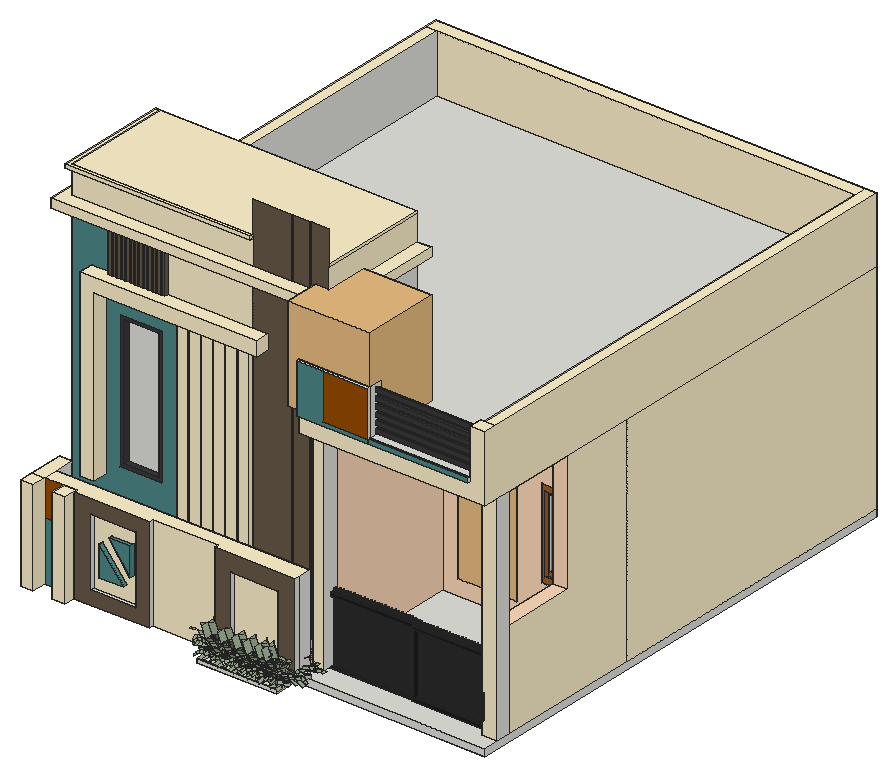
# SketchUp Ruby script. Lengths in inches.
U = 1.inch
M = Sketchup.active_model
def pt(a) = Geom::Point3d.new(a.map { |v| v * U })
def face(e, loops, mat)
  f = e.add_face(loops[0].map { |a| pt(a) })
  loops[1..].each { |l| e.add_face(l.map { |a| pt(a) }).erase! }
  f.material = f.back_material = mat if mat
  f
end
# faces: each face lists its corners as indices into pts; further lists are holes
def faces(e, pts, list, mat = nil) = list.each { |f| face(e, (f[0].is_a?(Array) ? f : [f]).map { |l| l.map { |i| pts[i] } }, mat) }
# xy, xz, yz: faces in a plane at the given z, y or x. An outline is a flat list of corners, or four numbers for a rectangle; further outlines are holes
def ring(l) = l.size == 4 ? [[l[0], l[1]], [l[2], l[1]], [l[2], l[3]], [l[0], l[3]]] : l.each_slice(2).to_a
def flat(e, list, mat, &to3) = list.each { |f| face(e, (f[0].is_a?(Array) ? f : [f]).map { |l| ring(l).map { |u, v| to3.(u, v) } }, mat) }
def xy(e, z, list, mat = nil) = flat(e, list, mat) { |x, y| [x, y, z] }
def xz(e, y, list, mat = nil) = flat(e, list, mat) { |x, z| [x, y, z] }
def yz(e, x, list, mat = nil) = flat(e, list, mat) { |y, z| [x, y, z] }
def lines(e, pts, list) = list.each { |a, b| e.add_line(pt(pts[a]), pt(pts[b])) }
# prism: a flat outline (further loops are holes) pulled along v
def prism(e, loops, v, mat = nil)
  f = face(e, loops, mat); d = Geom::Vector3d.new(v.map { |x| x * U })
  f.pushpull(f.normal.samedirection?(d) ? d.length : -d.length)
end
def box(e, o, s, mat = nil) = prism(e, [[o, [o[0] + s[0], o[1], o[2]], [o[0] + s[0], o[1] + s[1], o[2]], [o[0], o[1] + s[1], o[2]]]], [0, 0, s[2]], mat)
def at(x, y, z, deg = 0) = Geom::Transformation.translation(pt([x, y, z])) * Geom::Transformation.rotation(ORIGIN, Z_AXIS, deg.degrees)
def axes(o, x, y, z) = Geom::Transformation.new([*x, 0, *y, 0, *z, 0, *pt(o).to_a, 1])
def part(name) = M.definitions.add(name)
# library, detail: a bought-in or finely detailed component or shape, given as its bounding box
def library(name, o, s) = part(name).tap { |d| box(d.entities, o, s) }
def detail(e, o, s) = box(e.add_group.entities, o, s)
def put(e, d, t, mat = nil) = e.add_instance(d, t).tap { |i| i.material = mat if mat }
def group(e, t, mat = nil) = e.add_group.tap { |g| g.transformation = t; g.material = mat if mat }.entities
root = M.entities
M.materials.add("[Color C01]").color = [255, 219, 186]
M.materials.add("[Color C07]").color = [104, 89, 74]
M.materials.add("[Color C07]1").color = [153, 76, 0]
M.materials.add("[Color D01]").color = [255, 242, 204]
M.materials.add("[Color H08]").color = [77, 137, 137]
M.materials.add("[Color M07]").color = [58, 58, 58]
M.materials.add("[Color M08]").color = [30, 30, 30]
M.materials.add("[Translucent_Glass_Safety]").color = [204, 235, 244]
M.materials["[Translucent_Glass_Safety]"].alpha = 0.5
M.materials.add("[Translucent_Glass_Sky_Reflection]").color = [125, 138, 183]
M.materials["[Translucent_Glass_Sky_Reflection]"].alpha = 0.52
M.materials.add("[Wood Square Tile 01]").color = [164, 91, 44]
M.materials.add("[Wood Square Tile 02]").color = [160, 95, 34]
M.materials.add("hymenocallis littoralis").color = [156, 172, 146]
c1 = part("Group\#428")
prism(c1.entities,[[[0,1.97,0],[0,1.97,1.18],[0,0,1.18],[0,0,0]],[[0,1.92,1.13],[0,1.92,0.05],[0,0.05,0.05],[0,0.05,1.13]]],[98.43,0,0])
c2 = part("Group\#430")
xy(c2.entities,0,[[0.3,0,0.22,0.01,0.15,0.04,0.09,0.09,0.04,0.15,0.01,0.22,0,0.3,0.3,0.3],[0.3,0,0.3,0.3,0.59,0.3,0.58,0.22,0.55,0.15,0.5,0.09,0.44,0.04,0.37,0.01],[0,0.3,0.01,0.37,0.04,0.44,0.09,0.5,0.15,0.55,0.22,0.58,0.3,0.59,0.3,0.3],[0.3,0.3,0.3,0.59,0.37,0.58,0.44,0.55,0.5,0.5,0.55,0.44,0.58,0.37,0.59,0.3]])
xy(c2.entities,39.37,[[0.3,0,0.37,0.01,0.44,0.04,0.5,0.09,0.55,0.15,0.58,0.22,0.59,0.3,0.58,0.37,0.55,0.44,0.5,0.5,0.44,0.55,0.37,0.58,0.3,0.59,0.22,0.58,0.15,0.55,0.09,0.5,0.04,0.44,0.01,0.37,0,0.3,0.01,0.22,0.04,0.15,0.09,0.09,0.15,0.04,0.22,0.01]])
p = [[0.09,0.09,0],[0.15,0.04,0],[0.15,0.04,39.37],[0.09,0.09,39.37],[0.22,0.01,0],[0.22,0.01,39.37],
  [0.3,0,0],[0.3,0,39.37],[0.37,0.01,0],[0.37,0.01,39.37],[0.44,0.04,0],[0.44,0.04,39.37],
  [0.5,0.09,0],[0.5,0.09,39.37],[0.01,0.22,0],[0.04,0.15,0],[0.04,0.15,39.37],[0.01,0.22,39.37],
  [0.55,0.15,0],[0.55,0.15,39.37],[0.58,0.22,0],[0.58,0.22,39.37],[0,0.3,0],[0,0.3,39.37],
  [0.59,0.3,0],[0.59,0.3,39.37],[0.01,0.37,0],[0.01,0.37,39.37],[0.58,0.37,0],[0.58,0.37,39.37],
  [0.09,0.5,0],[0.04,0.44,0],[0.04,0.44,39.37],[0.09,0.5,39.37],[0.55,0.44,0],[0.5,0.5,0],
  [0.5,0.5,39.37],[0.55,0.44,39.37],[0.15,0.55,0],[0.15,0.55,39.37],[0.44,0.55,0],[0.44,0.55,39.37],
  [0.22,0.58,0],[0.22,0.58,39.37],[0.3,0.59,0],[0.3,0.59,39.37],[0.37,0.58,0],[0.37,0.58,39.37]]
faces(c2.entities,p,[[0,1,2,3],[1,4,5,2],[4,6,7,5],[6,8,9,7],[8,10,11,9],[10,12,13,11],[14,15,16,17],[15,0,3,16],
  [12,18,19,13],[18,20,21,19],[22,14,17,23],[20,24,25,21],[26,22,23,27],[24,28,29,25],[30,31,32,33],[31,26,27,32],
  [34,35,36,37],[28,34,37,29],[38,30,33,39],[35,40,41,36],[42,38,39,43],[44,42,43,45],[46,44,45,47],[40,46,47,41]])
c3 = part("Group\#429")
prism(c3.entities,[[[0.01,0.22,35.83],[0,0.3,35.83],[0.01,0.37,35.83],[0.04,0.44,35.83],[0.09,0.5,35.83],[0.15,0.55,35.83],[0.22,0.58,35.83],[0.3,0.59,35.83],[0.37,0.58,35.83],[0.44,0.55,35.83],[0.5,0.5,35.83],[0.55,0.44,35.83],[0.58,0.37,35.83],[0.59,0.3,35.83],[0.58,0.22,35.83],[0.55,0.15,35.83],[0.5,0.09,35.83],[0.44,0.04,35.83],[0.37,0.01,35.83],[0.3,0,35.83],[0.22,0.01,35.83],[0.15,0.04,35.83],[0.09,0.09,35.83],[0.04,0.15,35.83]]],[0,0,3.54])
c4 = part("Metal railing panel")
g1 = group(c4.entities,at(0,0,0))
put(g1,c1,axes([0,0,39.76],[1,0,0],[0,0,-1],[0,1,0]),"[Color M08]")
put(g1,c1,axes([0,0,1.97],[1,0,0],[0,0,-1],[0,1,0]),"[Color M08]")
put(g1,c1,axes([98.43,0,37.8],[0,0,-0.364],[-1,0,0],[0,1,0]),"[Color M08]")
put(g1,c1,axes([1.97,0,37.8],[0,0,-0.364],[-1,0,0],[0,1,0]),"[Color M08]")
g2 = group(c4.entities,at(1.67,0.3,1.97))
put(g2,c2,at(78.74,0,0),"[Color M08]")
put(g2,c2,at(90.55,0,0),"[Color M08]")
put(g2,c2,at(82.68,0,0),"[Color M08]")
put(g2,c2,at(86.61,0,0),"[Color M08]")
put(g2,c2,at(66.93,0,0),"[Color M08]")
put(g2,c2,at(11.8125,0,0),"[Color M08]")
put(g2,c2,at(15.75,0,0),"[Color M08]")
put(g2,c2,at(47.24,0,0),"[Color M08]")
put(g2,c2,at(59.06,0,0),"[Color M08]")
put(g2,c3,at(0,0,0),"[Color M08]")
put(g2,c2,at(39.37,0,0),"[Color M08]")
put(g2,c2,at(62.99,0,0),"[Color M08]")
put(g2,c2,at(55.12,0,0),"[Color M08]")
put(g2,c2,at(19.69,0,0),"[Color M08]")
put(g2,c2,at(35.43,0,0),"[Color M08]")
put(g2,c2,at(7.875,0,0),"[Color M08]")
put(g2,c2,at(23.62,0,0),"[Color M08]")
put(g2,c2,at(31.5,0,0),"[Color M08]")
put(g2,c2,at(43.31,0,0),"[Color M08]")
put(g2,c2,at(27.56,0,0),"[Color M08]")
put(g2,c2,at(3.9375,0,0),"[Color M08]")
put(g2,c2,at(51.18,0,0),"[Color M08]")
put(g2,c2,at(70.87,0,0),"[Color M08]")
put(g2,c2,at(74.8,0,0),"[Color M08]")
put(g2,c3,at(94.49,0,0),"[Color M08]")
c5 = part("Sliding window")
xy(c5.entities,0,[[0,0,4.33,55.51]])
xy(c5.entities,2.76,[[0,2.76,2,27.76],[0,27.76,0.82,52.76],[0.82,27.76,2.36,52.76]])
xy(c5.entities,2.76,[[3.15,2.76,4.33,27.76]],"[Wood Square Tile 01]")
xy(c5.entities,2.76,[[2.36,27.76,4.33,52.76]],"[Wood Square Tile 02]")
xy(c5.entities,4.72,[[2,4.72,2.4,26.38],[2.76,4.72,3.15,26.38],[0.82,29.13,1.22,50.79],[1.97,29.13,2.36,50.79]])
xy(c5.entities,36.61,[[2,4.72,2.4,26.38],[2.76,4.72,3.15,26.38],[0.82,29.13,1.22,50.79],[1.97,29.13,2.36,50.79]])
xy(c5.entities,38.58,[[0,2.76,2,27.76],[0,27.76,0.82,52.76],[0.82,27.76,2.36,52.76]])
xy(c5.entities,38.58,[[3.15,2.76,4.33,27.76],[2.36,27.76,4.33,52.76]],"[Wood Square Tile 01]")
xy(c5.entities,41.34,[[0,0,4.33,55.51]])
xz(c5.entities,0,[[0,0,4.33,41.34]])
xz(c5.entities,2.76,[[0,2.76,2,38.58]])
xz(c5.entities,2.76,[[3.15,2.76,4.33,38.58]],"[Wood Square Tile 01]")
xz(c5.entities,4.72,[[2,4.72,2.4,36.61],[2.76,4.72,3.15,36.61]])
xz(c5.entities,26.38,[[2,4.72,2.4,36.61],[2.76,4.72,3.15,36.61]])
xz(c5.entities,27.76,[[0.82,2.76,2,38.58],[2,2.76,2.36,38.58],[2.36,2.76,3.15,38.58]])
xz(c5.entities,29.13,[[0.82,4.72,1.22,36.61],[1.97,4.72,2.36,36.61]])
xz(c5.entities,50.79,[[0.82,4.72,1.22,36.61],[1.97,4.72,2.36,36.61]])
xz(c5.entities,52.76,[[0,2.76,0.82,38.58],[0.82,2.76,2.36,38.58]])
xz(c5.entities,52.76,[[2.36,2.76,4.33,38.58]],"[Wood Square Tile 01]")
xz(c5.entities,55.51,[[0,0,4.33,41.34]])
yz(c5.entities,0,[[[0,0,55.51,41.34],[2.76,2.76,52.76,38.58]]])
yz(c5.entities,0.82,[[[27.76,2.76,52.76,38.58],[29.13,4.72,50.79,36.61]]])
yz(c5.entities,1.22,[[29.13,4.72,50.79,36.61]],"[Translucent_Glass_Sky_Reflection]")
yz(c5.entities,1.97,[[29.13,4.72,50.79,36.61]],"[Translucent_Glass_Sky_Reflection]")
yz(c5.entities,2,[[[2.76,2.76,27.76,38.58],[4.72,4.72,26.38,36.61]]])
yz(c5.entities,2.36,[[[27.76,2.76,52.76,38.58],[29.13,4.72,50.79,36.61]]],"[Wood Square Tile 02]")
yz(c5.entities,2.4,[[4.72,4.72,26.38,36.61]],"[Translucent_Glass_Safety]")
yz(c5.entities,2.76,[[4.72,4.72,26.38,36.61]],"[Translucent_Glass_Safety]")
yz(c5.entities,3.15,[[[2.76,2.76,27.76,38.58],[4.72,4.72,26.38,36.61]]],"[Wood Square Tile 02]")
yz(c5.entities,4.33,[[[0,0,55.51,41.34],[2.76,2.76,52.76,38.58]]],"[Wood Square Tile 02]")
c6 = library("door2",[0,0,0],[35.42,7.875,78.74])
c7 = part("Group\#856")
xy(c7.entities,7.38,[[0,0,5.5,15.91]],"hymenocallis littoralis")
p = [[5.5,28.78,0],[5.5,26.79,3.44],[0,26.79,3.44],[0,28.78,0],[0,23.75,6],[5.5,23.75,6],
  [0,15.91,7.38],[5.5,15.91,7.38]]
faces(c7.entities,p,[[0,1,2,3],[4,2,1,5],[6,4,5,7]],"hymenocallis littoralis")
c8 = part("Group\#854")
xy(c8.entities,7.38,[[0,0,5.5,15.91],[0,15.91,5.5,23.87]],"hymenocallis littoralis")
p = [[5.5,31.07,4.3],[5.5,27.74,6.47],[0,27.74,6.47],[0,31.07,4.3],[0,23.87,7.38],[5.5,23.87,7.38]]
faces(c8.entities,p,[[0,1,2,3],[4,2,1,5]],"hymenocallis littoralis")
c9 = part("Group\#857")
xy(c9.entities,7.38,[[0,0,5.6,15.91]],"hymenocallis littoralis")
p = [[5.6,28.78,0],[5.6,26.79,3.44],[0,26.79,3.44],[0,28.78,0],[0,23.75,6],[5.6,23.75,6],
  [0,15.91,7.38],[5.6,15.91,7.38]]
faces(c9.entities,p,[[0,1,2,3],[4,2,1,5],[6,4,5,7]],"hymenocallis littoralis")
c10 = part("Group\#855")
put(c10.entities,c8,axes([6.09,8.57,-0.52],[0.446,0.85617,0.26089],[-0.18444,-0.19731,0.96283],[0.87582,-0.47754,0.0699]))
put(c10.entities,c8,axes([6.29,7.28,-1.71],[0.37058,0.92707,-0.05667],[-0.32382,0.19004,0.99128],[0.87712,-0.32925,0.34964]))
put(c10.entities,c8,axes([11.04,16.14,-0.7],[1,0,0],[0,0.16628,1.02662],[0,-1.18456,0.19186]))
c11 = part("Group\#860")
put(c11.entities,c7,axes([24.57,32.05,-1.76],[0.9552,-0.22102,-0.19681],[0.4036,0.95545,0.88585],[-0.00568,-0.67859,0.7345]))
put(c11.entities,c7,axes([23.95,29.24,-2.4],[0,1,0],[-0.76041,0,0.64945],[0.64945,0,0.76041]))
put(c11.entities,c7,axes([24.22,24.72,-0.48],[-0.70711,0.70711,0],[-0.32757,-0.32757,0.80237],[0.61237,0.61237,0.5]))
put(c11.entities,c8,axes([20.66,37.22,-0.63],[1.12361,0.03262,0.39091],[-0.43499,0.29739,0.78777],[0.09852,-1.27434,0.37535]))
put(c11.entities,c7,axes([28.75,24.45,-2.4],[-1,0,0],[0,-0.76041,0.64945],[0,0.64945,0.76041]))
put(c11.entities,c9,axes([30.4,30.98,-3.7],[0.65676,-0.72002,0.22414],[0.55667,0.66341,0.5],[-0.50871,-0.20361,0.83652]))
put(c11.entities,c9,axes([32.41,29.61,-3.7],[0.04029,-0.97372,0.22414],[0.85287,0.15038,0.5],[-0.52057,0.17102,0.83652]))
put(c11.entities,c7,axes([31.89,25.85,-1.76],[-0.92056,0.33739,-0.19681],[-0.5186,-0.89824,0.88585],[0.08952,0.67268,0.7345]))
put(c11.entities,c7,axes([25.55,34.78,-0.48],[0.86603,0.5,0],[-0.25,0.43301,0.86603],[0.43301,-0.75,0.5]))
put(c11.entities,c9,axes([20.4,16.9375,-8.07],[-0.70711,0.70711,0],[-0.35754,-0.35754,0.65422],[1.3987,1.3987,1.52882]))
put(c11.entities,c7,axes([32.86,34.14,-0.48],[0.76604,-0.64279,0],[0.32139,0.38302,0.86603],[-0.55667,-0.66341,0.5]))
put(c11.entities,c7,axes([27.15,34.7,-0.1],[0.82472,-0.17528,-0.53769],[0.53769,0.53769,0.64945],[0.17528,-0.82472,0.53769]))
put(c11.entities,c7,axes([33.58,28.77,-2.4],[0,-1,0],[0.76041,0,0.64945],[-0.64945,0,0.76041]))
put(c11.entities,c7,axes([26.43,23.87,-2.81],[-0.75126,0.04415,0.65853],[0.53769,-0.53769,0.64945],[0.38276,0.84199,0.3802]))
put(c11.entities,c7,axes([28.78,23.98,-2.4],[-1,0,0],[0,-0.76041,0.64945],[0,0.64945,0.76041]))
put(c11.entities,c7,axes([25.39,25.38,-2.4],[-0.70711,0.70711,0],[-0.53769,-0.53769,0.64945],[0.45923,0.45923,0.76041]))
put(c11.entities,c7,axes([27.32,21.63,-0.1],[-0.45923,0.70711,-0.53769],[-0.76041,0,0.64945],[0.45923,0.70711,0.53769]))
put(c11.entities,c7,axes([25.17,27.625,-1.76],[0.56416,0.80187,-0.19681],[-0.66673,0.66673,0.80532],[0.62659,-0.26057,0.7345]))
put(c11.entities,c9,axes([27.59,27.04,-3.96],[-0.8993,-0.06127,0.43301],[0.2962,-0.8138,0.5],[0.32175,0.57791,0.75]))
put(c11.entities,c9,axes([26.98,24.5,-3.18],[-0.5,0.86603,0],[-0.75,-0.43301,0.5],[0.43301,0.25,0.86603]))
put(c11.entities,c9,axes([24.55,27.74,-3.7],[0.29517,0.92878,0.22414],[-0.85287,0.15038,0.5],[0.43068,-0.33875,0.83652]))
put(c11.entities,c9,axes([24.26,29.8,-3.18],[0.76604,0.64279,0],[-0.47317,0.5639,0.425],[0.32139,-0.38302,0.86603]))
put(c11.entities,c9,axes([25.98,32.46,-3.18],[1,0,0],[0,0.86603,0.5],[0,-0.5,0.86603]))
put(c11.entities,c7,axes([28.78,33.57,-2.4],[1,0,0],[0,0.76041,0.64945],[0,-0.64945,0.76041]))
put(c11.entities,c10,at(14.99,21.38,2.5))
put(c11.entities,c8,axes([34.63,26.34,-1.46],[-0.70089,-0.70877,0.07994],[0.4756,-0.38088,0.79293],[-0.53156,0.59378,0.60405]))
put(c11.entities,c8,axes([28.14,16.92,1.8125],[-1.19719,0.6912,0],[-0.09607,-0.16641,0.94244],[0.68444,1.18549,0.17613]))
put(c11.entities,c8,axes([31.5625,35.84,0.97],[0.66765,-1.1564,0.35779],[0.04445,0.30732,0.91033],[-1.20828,-0.64496,0.17012]))
put(c11.entities,c8,axes([38.94,22.51,0.89],[-0.97932,-0.67164,-0.05202],[0.27787,-0.41401,0.90999],[-0.85985,0.93577,0.32097]))
put(c11.entities,c8,axes([38.44,21.09,1.98],[-1.02864,-0.54856,0.2395],[0.33481,0.06999,0.88388],[-0.77261,1.08328,0.06417]))
put(c11.entities,c9,axes([35.02,30.51,-1.3],[-0.17365,-0.98481,0],[0.60224,-0.10619,0.79122],[-0.7792,0.13739,0.61153]))
put(c11.entities,c9,axes([29.41,22.33,-1.3],[-0.93969,0.34202,0],[-0.20915,-0.57465,0.79122],[0.27061,0.74351,0.61153]))
put(c11.entities,c8,axes([19.64,36,-1.62],[1.18194,0.09546,0.08234],[-0.14377,0.68823,0.76313],[0.21457,-1.1326,0.62386]))
put(c11.entities,c9,axes([24.25,24.14,-1.3],[-0.34202,0.93969,0],[-0.57465,-0.20915,0.79122],[0.74351,0.27061,0.61153]))
put(c11.entities,c9,axes([25.98,34.61,-1.3],[1,0,0],[0,0.61153,0.79122],[0,-0.79122,0.61153]))
put(c11.entities,c9,axes([31.16,34.41,-1.64],[0.56518,-0.80224,-0.19234],[0.73413,0.34233,0.72935],[-0.47639,-0.50772,0.71782]))
put(c11.entities,c9,axes([40.52,26.84,-5.82],[-0.42262,-0.90631,0],[0.48019,-0.22391,0.68552],[-1.43418,0.66877,1.22305]))
put(c11.entities,c7,axes([29.86,38.42,-1.01],[0.89064,-0.37013,0.26413],[-0.03924,0.63286,1.01918],[-0.45353,-0.76487,0.45748]))
put(c11.entities,c7,axes([29.34,22.4,-0.48],[-0.99619,-0.08716,0],[0.04358,-0.4981,0.86603],[-0.07548,0.86273,0.5]))
c12 = part("Group\#858")
xz(c12.entities,10.07,[[9.07,0,10.07,31.01],[0,31.01,0,45.12,20.13,45.12,20.13,31.01,10.07,31.01,10.07,32.58,9.07,32.58,9.07,31.01]],"hymenocallis littoralis")
yz(c12.entities,10.07,[[0,31.01,20.13,45.12]],"hymenocallis littoralis")
p = [[9.57,9.2,0],[10.07,10.07,0],[10.07,10.07,31.01],[10.07,10.07,32.58],[9.57,9.2,32.58]]
faces(c12.entities,p,[[0,1,2,3,4]],"hymenocallis littoralis")
c13 = part("cây lá nắng")
put(c13.entities,c11,axes([49.26,-2.75,0],[0.63109,0.63109,0],[-0.63109,0.63109,0],[0,0,0.935]))
g3 = group(c13.entities,at(26.6,-8.68,0))
put(g3,c7,axes([-4.72,35.73,-1.65],[0.74231,0.46334,-0.18402],[-0.34827,0.85768,0.82827],[0.42467,-0.43184,0.68675]))
put(g3,c7,axes([-3.34,33.57,-2.24],[-0.63109,0.63109,0],[-0.47989,-0.47989,0.60723],[0.40986,0.40986,0.71098]))
put(g3,c7,axes([-0.3125,30.89,-0.45],[-0.8925,0,0],[0,-0.41345,0.75022],[0,0.77293,0.4675]))
put(g3,c8,axes([-10.79,39.66,-0.59],[0.68852,0.72969,0.3655],[-0.4622,-0.08684,0.73657],[0.86641,-0.74205,0.35095]))
put(g3,c7,axes([2.71,33.57,-2.24],[-0.63109,-0.63109,0],[0.47989,-0.47989,0.60723],[-0.40986,0.40986,0.71098]))
put(g3,c9,axes([-0.37,38.74,-3.46],[0.86887,-0.03992,0.20957],[-0.06737,0.76999,0.4675],[-0.19255,-0.44954,0.78214]))
put(g3,c9,axes([1.76,39.14,-3.46],[0.63993,-0.58908,0.20957],[0.44333,0.63315,0.4675],[-0.43646,-0.2206,0.78214]))
put(g3,c7,axes([3.81,36.4375,-1.65],[-0.79389,-0.36803,-0.18402],[0.23959,-0.89415,0.82827],[-0.36803,0.48102,0.68675]))
put(g3,c7,axes([-5.83,38.07,-0.45],[0.231,0.86209,0],[-0.43104,0.1155,0.80973],[0.74659,-0.20005,0.4675]))
put(g3,c9,axes([2.18,23.5625,-7.55],[-0.8925,0,0],[0,-0.45128,0.6117],[0,1.76542,1.42944]))
put(g3,c7,axes([-0.8125,42.28,-0.45],[0.8891,0.07779,0],[-0.03889,0.44455,0.80973],[0.06737,-0.76999,0.4675]))
put(g3,c7,axes([-4.76,39.03,-0.09],[0.63109,0.40986,-0.50274],[0,0.67866,0.60723],[0.63109,-0.40986,0.50274]))
put(g3,c7,axes([3.03,39.35,-2.24],[0.63109,-0.63109,0],[0.47989,0.47989,0.60723],[-0.40986,-0.40986,0.71098]))
put(g3,c7,axes([1.61,31.74,-2.625],[-0.50198,-0.44625,0.61573],[0.67866,0,0.60723],[-0.28982,0.77293,0.35549]))
put(g3,c7,axes([3.03,33.3,-2.24],[-0.63109,-0.63109,0],[0.47989,-0.47989,0.60723],[-0.40986,0.40986,0.71098]))
put(g3,c7,axes([0.01,32.04,-2.24],[-0.8925,0,0],[0,-0.67866,0.60723],[0,0.57963,0.71098]))
put(g3,c7,axes([3.59,30.89,-0.09],[-0.73607,0.15643,-0.50274],[-0.47989,-0.47989,0.60723],[-0.15643,0.73607,0.50274]))
put(g3,c7,axes([-1.55,33.32,-1.65],[-0.15002,0.86209,-0.18402],[-0.84154,0,0.75297],[0.55988,0.231,0.68675]))
put(g3,c9,axes([0.35,34.48,-3.71],[-0.52887,-0.60621,0.40487],[0.70051,-0.32665,0.4675],[-0.16166,0.56777,0.70125]))
put(g3,c9,axes([2.61,39.13,-1.74],[-0.86209,0.231,0],[-0.23031,-0.85954,0.15531],[0.03162,0.11799,0.91645]))
put(g3,c9,axes([-2.02,33,-3.46],[-0.39986,0.77243,0.20957],[-0.63315,-0.44333,0.4675],[0.48558,0.05802,0.78214]))
put(g3,c9,axes([-3.49,34.12,-2.97],[0.07779,0.8891,0],[-0.65449,0.05726,0.39737],[0.44455,-0.03889,0.80973]))
put(g3,c9,axes([-4.09,36.88,-2.97],[0.63109,0.63109,0],[-0.54654,0.54654,0.4675],[0.31555,-0.31555,0.80973]))
put(g3,c7,axes([-3.02,39.35,-2.24],[0.63109,0.63109,0],[-0.47989,0.47989,0.60723],[0.40986,-0.40986,0.71098]))
put(g3,c10,axes([-4.03,22.95,2.33],[0.63109,0.63109,0],[-0.63109,0.63109,0],[0,0,0.935]))
put(g3,c8,axes([5.24,38.48,-1.37],[0.00497,-0.88963,0.07474],[0.54052,0.05978,0.74139],[-0.71019,0.03927,0.56479]))
put(g3,c8,axes([7.08,28.4375,1.7],[-1.19175,-0.31933,0],[0.04439,-0.16565,0.88118],[-0.31621,1.1801,0.16468]))
put(g3,c8,axes([-2.7,42.54,0.91],[1.15114,-0.30845,0.33454],[-0.1659,0.22199,0.85115],[-0.3555,-1.16957,0.15907]))
put(g3,c8,axes([10.37,38.78,0.83],[-0.19417,-1.04191,-0.04864],[0.43664,-0.08592,0.85084],[-1.1332,0.04791,0.30011]))
put(g3,c8,axes([10.95,37.5625,1.85],[-0.30298,-0.99536,0.22393],[0.16713,0.25547,0.82643],[-1.17124,0.19607,0.06]))
put(g3,c9,axes([2.84,41.36,-1.22],[0.51192,-0.73109,0],[0.44708,0.31305,0.73979],[-0.57846,-0.40504,0.57178]))
put(g3,c9,axes([4.47,32.65,-1.22],[-0.80888,-0.37719,0],[0.23066,-0.49465,0.73979],[-0.29844,0.64,0.57178]))
put(g3,c8,axes([-10.32,35.12,-1.51],[0.68567,0.80616,0.07699],[-0.52507,0.3436,0.71352],[0.85019,-0.57936,0.58331]))
put(g3,c9,axes([0.07,30.54,-1.22],[-0.80888,0.37719,0],[-0.23066,-0.49465,0.73979],[0.29844,0.64,0.57178]))
put(g3,c9,axes([-5.45,38.24,-1.22],[0.63109,0.63109,0],[-0.38593,0.38593,0.73979],[0.49934,-0.49934,0.57178]))
put(g3,c9,axes([-2.05,41.38,-1.53],[0.86296,-0.14961,-0.17984],[0.24726,0.67935,0.68194],[0.01977,-0.62107,0.67116]))
put(g3,c9,axes([8.63,42.51,-5.4375],[0.30525,-0.83868,0],[0.44435,0.16173,0.64096],[-1.32716,-0.48305,1.14356]))
put(g3,c7,axes([-5.4,43.09,-0.94],[0.79566,0.32849,0.24696],[-0.42416,0.37462,0.95293],[0.19648,-0.76892,0.42774]))
put(g3,c7,axes([4.38,32.65,-0.45],[-0.57369,-0.68369,0],[0.34185,-0.28684,0.80973],[-0.5921,0.49683,0.4675]))
put(g3,c9,axes([-2,33.84,-0.15],[-0.24601,0.85793,0],[-0.85539,-0.24528,0.15531],[0.11742,0.03367,0.91645]))
put(g3,c9,axes([0.17,30.83,-4.47],[-0.24601,0.85793,0],[-0.85539,-0.24528,0.15531],[0.11742,0.03367,0.91645]))
put(g3,c9,axes([-1.97,32.18,-4.47],[0.58524,0.67383,0],[-0.67184,0.58351,0.15531],[0.09222,-0.0801,0.91645]))
put(g3,c9,axes([-2,34.71,-4.47],[0.88392,-0.12346,0],[0.12309,0.88131,0.15531],[-0.0169,-0.12098,0.91645]))
put(g3,c9,axes([0.11,36.12,-4.47],[0.37822,-0.8084,0],[0.80601,0.37711,0.15531],[-0.11064,-0.05177,0.91645]))
put(c13.entities,c12,axes([29.71,14.29,6.94],[0.425,0.73612,0],[-0.6771,0.39092,-0.33349],[-0.26859,0.15507,0.72712]))
put(c13.entities,c12,axes([42.0625,26.12,6.94],[0.85,0,0],[0,0.78185,-0.33349],[0,0.33349,0.78185]))
put(c13.entities,c11,axes([7.3125,23.0625,0],[0.8925,0,0],[0,0.8925,0],[0,0,0.935]))
put(c13.entities,c12,axes([24.4375,40.23,2.05],[0.85,0,0],[0,0.85,0],[0,0,0.85]))
c14 = part("Planting+101")
put(c14.entities,c13,axes([21.34,32.96,-4.59],[0,-0.71,0],[-0.71,0,0],[0,0,0.71]))
c15 = library("Flora+17",[-57.52,158.6,-38.64],[66.99,62.88,77.28])
c16 = part("Group\#1")
xz(c16.entities,0,[[0,0,2.8125,38.62]])
yz(c16.entities,0,[[0,0,3,38.62]])
yz(c16.entities,2.8125,[[0,0,3,38.62]])
c17 = part("Group\#2")
p = [[0,0,0.02],[0,1.98,0],[81.3125,1.98,0],[81.3125,0,0.02],[0,0.12,3.625],[81.3125,0.12,3.625],
  [0,2.11,3.61],[81.3125,2.11,3.61]]
faces(c17.entities,p,[[0,1,2,3],[4,0,3,5],[1,6,7,2],[6,4,5,7]])
xy(root,0,[[150.35,2.54,150.35,21.8125,151.875,21.8125,151.875,4.0625,213.72,4.0625,213.72,19.97,215.25,19.97,215.25,2.54],[151.875,4.0625,213.72,18.4375],[0,9.8125,10.625,21.8125],[26.125,9.8125,36.75,21.8125],[36.75,18.4375,36.75,21.8125,0,21.8125,0,49.6875,10.625,49.6875,10.625,421.6875,370.625,421.6875,370.625,21.8125,217.88,21.8125,217.88,19.97,151.875,19.97,151.875,21.8125,98.84,21.8125,98.84,18.4375],
  [151.875,18.4375,213.72,19.97]])
xy(root,2.4375,[[150.35,2.54,215.25,2.54,215.25,18.4375,213.72,18.4375,213.72,4.0625,151.875,4.0625,151.875,21.8125,150.35,21.8125],[213.72,18.4375,215.25,19.97],[215.25,18.4375,217.88,19.97]])
xy(root,6,[[217.88,21.8125,370.625,21.8125,370.625,33.85,358.42,33.85,358.42,166.35,220.5,166.35,220.5,49.6875,227.12,49.6875,227.12,36.0625,217.88,36.0625,217.88,49.6875,205.92,49.6875,205.92,49.99,205.0625,49.99,205.0625,49.6875,190.92,49.6875,190.92,49.99,190,49.99,190,49.6875,158.1875,49.6875,158.1875,49.99,157.79,49.99,157.79,46.6875,148.18,46.6875,148.18,49.99,147.78,49.99,147.78,46.6875,138.17,46.6875,138.17,49.99,137.77,49.99,137.77,46.6875,128.17,46.6875,128.17,49.99,127.77,49.99,127.77,46.6875,118.16,46.6875,118.16,49.99,117.76,49.99,117.76,46.6875,108.15,46.6875,108.15,49.99,107.75,49.99,107.75,46.6875,98.15,46.6875,98.15,49.99,97.75,49.99,97.75,49.6875,10.625,49.6875,10.625,33.52,217.88,33.52],[358.42,45.67,370.625,166.35]])
xy(root,11.33,[[50.83,18.4375,87.51,21.8125]])
xy(root,13.49,[[165.37,18.4375,203.85,21.8125]])
xy(root,18,[[232.5,166.35,280.5,182.35]])
xy(root,22.6875,[[57.52,18.4375,77.7,21.8125]],"[Color H08]")
xy(root,39.88,[[301.46,166.35,353.08,191.72]])
xy(root,54.51,[[65.13,18.4375,83.06,21.8125]],"[Color H08]")
xy(root,64.51,[[165.37,18.4375,200.1875,21.8125],[200.1875,18.4375,203.85,21.8125]])
xy(root,66.67,[[50.83,18.4375,87.51,21.8125]])
xy(root,78,[[26.3125,37.6875,38.11,49.6875]])
xy(root,78,[[0,9.8125,10.625,21.8125],[26.125,9.8125,36.75,21.8125],[36.75,18.4375,98.84,18.4375,98.84,21.8125,151.875,21.8125,151.875,18.4375,217.88,18.4375,217.88,33.52,10.625,33.52,10.625,21.8125,36.75,21.8125],[0,21.8125,10.625,49.6875]],"[Color D01]")
xy(root,85.5625,[[358.42,45.67,370.625,106.01]],"[Color C01]")
xy(root,90.54,[[52.42,49.6875,81.72,54.8125]],"[Color M07]")
xy(root,102,[[232.5,166.35,280.5,182.35]])
xy(root,112.7,[[301.46,166.35,353.08,191.72]])
xy(root,183.5625,[[217.88,21.8125,217.88,49.6875,220.5,49.6875,220.5,166.35,358.42,166.35,358.42,106.01,370.625,106.01,370.625,45.67,358.42,45.67,358.42,33.85,370.625,33.85,370.625,21.8125]],"[Color C01]")
xy(root,184.3125,[[217.88,36.0625,227.12,49.6875]])
xy(root,189.9375,[[227.62,32.9375,361.5625,32.9375,361.5625,411.0625,19.625,411.0625,19.625,139.5,220.5,139.5,220.5,60.625,227.62,60.625]])
xy(root,196.53,[[52.42,49.6875,81.72,54.8125]],"[Color M07]")
xy(root,196.64,[[217.88,19.69,276.48,21.8]])
xy(root,200.25,[[276.48,21.8125,357.8,32.9375]])
xy(root,215.64,[[38.11,37.6875,38.11,49.6875,97.75,49.6875,97.75,49.99,98.15,49.99,98.15,46.6875,107.75,46.6875,107.75,49.99,108.15,49.99,108.15,46.6875,117.76,46.6875,117.76,49.99,118.16,49.99,118.16,46.6875,127.77,46.6875,127.77,49.99,128.17,49.99,128.17,46.6875,137.77,46.6875,137.77,49.99,138.17,49.99,138.17,46.6875,147.78,46.6875,147.78,49.99,148.18,49.99,148.18,46.6875,157.79,46.6875,157.79,49.99,158.1875,49.99,158.1875,49.6875,170.9375,49.6875,170.9375,37.6875]],"[Color D01]")
xy(root,227.33,[[26.3125,37.6875,170.9375,37.6875,170.9375,49.6875,45.2,49.6875,45.2,46.6875,42.38,46.6875,42.38,49.6875,26.3125,49.6875]],"[Color D01]")
xy(root,237.5625,[[217.88,19.69,276.48,21.8]])
xy(root,237.5625,[[217.88,21.8125,276.48,21.8125,276.48,32.9375,227.62,32.9375,227.62,60.625,220.5,60.625,220.5,49.6875,217.88,49.6875],[357.8,21.8125,370.625,32.9375],[361.5625,32.9375,370.625,421.6875],[10.625,139.5,19.625,411.0625],[10.625,411.0625,361.5625,421.6875]],"[Color D01]")
xy(root,265.94,[[158.1875,37.6875,158.1875,49.6875,190,49.6875,190,49.99,190.92,49.99,190.92,49.6875,205.0625,49.6875,205.0625,49.99,205.92,49.99,205.92,49.6875,220.5,49.6875,220.5,139.5,232.5,139.5,232.5,37.6875]])
xy(root,265.94,[[2.625,37.6875,2.625,139.5,10.625,139.5,10.625,49.6875,42.38,49.6875,42.38,46.6875,45.2,46.6875,45.2,49.6875,158.1875,49.6875,158.1875,37.6875]],"[Color D01]")
xy(root,272.92,[[2.625,37.6875,232.5,37.6875,232.5,139.5,220.5,139.5,220.5,49.6875,205.92,49.6875,205.92,49.99,205.0625,49.99,205.0625,49.6875,190.92,49.6875,190.92,49.99,190,49.99,190,49.6875,10.625,49.6875,10.625,139.5,2.625,139.5]],"[Color D01]")
xy(root,292.71,[[7.25,46.6875,10.625,49.6875],[10.625,46.6875,158.1875,49.6875],[7.25,49.6875,10.625,139.5]],"[Color D01]")
xy(root,292.96,[[158.1875,50.875,220.5,139.5]])
xy(root,295.71,[[7.25,46.6875,158.1875,46.6875,158.1875,49.6875,10.625,49.6875,10.625,139.5,7.25,139.5],[10.625,49.6875,158.1875,49.6875,158.1875,50.875,220.5,50.875,220.5,139.5,10.625,139.5]],"[Color D01]")
xy(root,321.41,[[190,49.6875,190.92,49.99],[205.0625,49.6875,205.92,49.99]])
xz(root,2.54,[[150.35,0,215.25,2.4375]])
xz(root,4.0625,[[151.875,0,213.72,2.4375]])
xz(root,9.8125,[[0,0,10.625,78],[26.125,0,36.75,78]],"[Color D01]")
xz(root,18.4375,[[[36.75,0,98.84,78],[50.83,11.33,87.51,66.67]],[[151.875,0,213.72,0,213.72,2.4375,217.88,2.4375,217.88,78,151.875,78],[165.37,13.49,203.85,64.51]]],"[Color C07]")
xz(root,18.4375,[[57.52,22.6875,77.7,22.6875,57.52,47.2],[83.06,31.32,83.06,54.51,65.13,54.51]],"[Color H08]")
xz(root,19.69,[[239.3,200.23,276.48,237.5625]],"[Color C07]1")
xz(root,19.69,[[217.88,196.64,276.48,196.64,276.48,200.23,239.3,200.23,239.3,237.5625,217.88,237.5625]],"[Color H08]")
xz(root,19.97,[[213.72,0,215.25,2.4375],[215.25,0,217.88,2.4375]])
xz(root,21.8,[[217.88,196.64,276.48,200.23],[217.88,200.23,276.48,237.5625]])
xz(root,21.8125,[[0,0,10.625,78],[26.125,0,36.75,78],[217.88,0,370.625,6]])
xz(root,21.8125,[[10.625,48.75,26.125,78]],"[Color C07]1")
xz(root,21.8125,[[98.84,0,150.35,0,150.35,2.4375,151.875,2.4375,151.875,78,98.84,78],[[50.83,11.33,87.51,66.67],[57.52,22.6875,57.52,47.2,77.7,22.6875],[83.06,31.32,65.13,54.51,83.06,54.51]],[165.37,13.49,203.85,64.51],[217.88,183.5625,370.625,183.5625,370.625,237.5625,357.8,237.5625,357.8,200.25,276.48,200.25,276.48,237.5625,217.88,237.5625]],"[Color D01]")
xz(root,21.8125,[[10.625,0,26.125,48.75]],"[Color H08]")
xz(root,32.9375,[[227.62,189.9375,227.62,237.5625,276.48,237.5625,276.48,200.25,357.8,200.25,357.8,237.5625,361.5625,237.5625,361.5625,189.9375]])
xz(root,33.52,[[10.625,6,206.03,78],[206.03,6,217.88,78]])
xz(root,33.85,[[358.42,6,370.625,183.5625]],"[Color D01]")
xz(root,36.0625,[[217.88,6,227.12,184.3125]],"[Color D01]")
xz(root,37.6875,[[26.3125,78,38.11,78,38.11,215.64,170.9375,215.64,170.9375,227.33,26.3125,227.33],[2.625,265.94,232.5,272.92]],"[Color D01]")
xz(root,45.67,[[358.42,6,370.625,85.5625],[358.42,85.5625,370.625,183.5625]])
xz(root,46.6875,[[98.15,6,107.75,215.64],[108.15,6,117.76,215.64],[118.16,6,127.77,215.64],[128.17,6,137.77,215.64],[138.17,6,147.78,215.64],
  [148.18,6,157.79,215.64],[7.25,292.71,158.1875,295.71]],"[Color D01]")
xz(root,49.6875,[[0,0,10.625,6],[0,6,10.625,78],[220.5,6,220.5,183.5625,217.88,183.5625,217.88,184.3125,227.12,184.3125,227.12,6],[217.88,189.5625,220.5,237.5625],[45.2,227.33,88.24,265.94],
  [10.625,292.71,158.1875,295.71]])
xz(root,49.6875,[[158.1875,6,190,6,190,265.94,158.1875,265.94,158.1875,227.33,170.9375,227.33,170.9375,215.64,158.1875,215.64],[190.92,6,205.0625,265.94],[205.92,6,217.88,6,217.88,237.5625,220.5,237.5625,220.5,265.94,205.92,265.94],[158.1875,272.92,190,321.41],[190.92,272.92,205.0625,321.41],
  [205.92,272.92,220.5,321.41]],"[Color C07]")
xz(root,49.6875,[[88.24,227.33,158.1875,265.94],[10.625,272.92,158.1875,292.71]],"[Color D01]")
xz(root,49.6875,[[[10.625,6,97.75,6,97.75,215.64,38.11,215.64,38.11,78,26.3125,78,26.3125,227.33,42.38,227.33,42.38,265.94,10.625,265.94],[49.35,87.47,84.79,199.6]]],"[Color H08]")
xz(root,49.6875,[[[49.35,87.47,84.79,199.6],[52.42,90.54,81.72,196.53]]],"[Color M07]")
xz(root,49.99,[[97.75,6,98.15,215.64],[107.75,6,108.15,215.64],[117.76,6,118.16,215.64],[127.77,6,128.17,215.64],[137.77,6,138.17,215.64],
  [147.78,6,148.18,215.64],[157.79,6,158.1875,215.64],[190,6,190.92,265.94],[205.0625,6,205.92,265.94],[190,272.92,190.92,321.41],
  [205.0625,272.92,205.92,321.41]])
xz(root,50.875,[[158.1875,292.96,220.5,295.71]])
xz(root,54.8125,[[52.42,90.54,81.72,196.53]])
xz(root,60.625,[[220.5,189.9375,227.62,237.5625]])
xz(root,106.01,[[358.42,85.5625,370.625,183.5625]],"[Color C01]")
xz(root,139.5,[[19.625,189.9375,19.625,237.5625,10.625,237.5625,10.625,295.71,220.5,295.71,220.5,189.9375],[2.625,265.94,10.625,272.92],[220.5,265.94,232.5,272.92],[7.25,292.71,10.625,295.71]],"[Color D01]")
xz(root,166.35,[[[220.5,6,358.42,183.5625],[232.5,18,280.5,102],[301.46,39.88,353.08,112.7]]],"[Color C01]")
xz(root,182.35,[[232.5,18,280.5,102]])
xz(root,191.72,[[301.46,39.88,353.08,112.7]])
xz(root,411.0625,[[19.625,189.9375,361.5625,237.5625]],"[Color D01]")
xz(root,421.6875,[[10.625,0,370.625,183.5625],[10.625,183.5625,370.625,237.5625]],"[Color D01]")
yz(root,0,[[9.8125,0,21.8125,78],[21.8125,0,49.6875,78]],"[Color D01]")
yz(root,2.625,[[37.6875,265.94,139.5,272.92]],"[Color D01]")
yz(root,7.25,[[46.6875,292.71,139.5,295.71]],"[Color D01]")
yz(root,10.625,[[33.52,6,49.6875,78],[49.6875,292.71,139.5,295.71]])
yz(root,10.625,[[9.8125,0,21.8125,78],[49.6875,0,421.6875,183.5625],[49.6875,183.5625,49.6875,189.5625,139.5,189.5625,139.5,237.5625,421.6875,237.5625,421.6875,183.5625],[49.6875,189.5625,139.5,265.94],[49.6875,272.92,139.5,292.71]],"[Color D01]")
yz(root,19.625,[[139.5,189.9375,411.0625,237.5625]])
yz(root,26.125,[[9.8125,0,21.8125,78]])
yz(root,26.3125,[[37.6875,78,49.6875,227.33]],"[Color D01]")
yz(root,36.75,[[18.4375,0,21.8125,78]])
yz(root,36.75,[[9.8125,0,18.4375,78]],"[Color D01]")
yz(root,38.11,[[37.6875,78,49.6875,215.64]],"[Color D01]")
yz(root,50.83,[[18.4375,11.33,21.8125,66.67]])
yz(root,52.42,[[49.6875,90.54,54.8125,196.53]],"[Color M07]")
yz(root,57.52,[[18.4375,22.6875,21.8125,47.2]],"[Color H08]")
yz(root,81.72,[[49.6875,90.54,54.8125,196.53]],"[Color M07]")
yz(root,83.06,[[18.4375,31.32,21.8125,54.51]],"[Color H08]")
yz(root,87.51,[[18.4375,11.33,21.8125,66.67]])
yz(root,97.75,[[49.6875,6,49.99,215.64]])
yz(root,98.15,[[46.6875,6,49.99,215.64]],"[Color D01]")
yz(root,98.84,[[18.4375,0,21.8125,78]])
yz(root,107.75,[[46.6875,6,49.99,215.64]])
yz(root,108.15,[[46.6875,6,49.99,215.64]])
yz(root,117.76,[[46.6875,6,49.99,215.64]])
yz(root,118.16,[[46.6875,6,49.99,215.64]])
yz(root,127.77,[[46.6875,6,49.99,215.64]])
yz(root,128.17,[[46.6875,6,49.99,215.64]])
yz(root,137.77,[[46.6875,6,49.99,215.64]])
yz(root,138.17,[[46.6875,6,49.99,215.64]])
yz(root,147.78,[[46.6875,6,49.99,215.64]])
yz(root,148.18,[[46.6875,6,49.99,215.64]])
yz(root,150.35,[[2.54,0,21.8125,2.4375]])
yz(root,151.875,[[4.0625,0,18.4375,2.4375],[18.4375,0,21.8125,2.4375],[18.4375,2.4375,21.8125,78]])
yz(root,157.79,[[46.6875,6,49.99,215.64]],"[Color D01]")
yz(root,158.1875,[[49.6875,6,49.99,215.64],[46.6875,292.71,49.6875,292.96],[49.6875,292.96,50.875,295.71]])
yz(root,158.1875,[[46.6875,292.96,49.6875,295.71]],"[Color D01]")
yz(root,165.37,[[18.4375,13.49,21.8125,64.51]])
yz(root,170.9375,[[37.6875,215.64,49.6875,227.33]],"[Color D01]")
yz(root,190,[[49.6875,6,49.99,265.94],[49.6875,272.92,49.99,321.41]])
yz(root,190.92,[[49.6875,6,49.99,183.5625],[49.6875,183.5625,49.99,189.5625],[49.6875,189.5625,49.99,237.5625],[49.6875,237.5625,49.99,265.94],[49.6875,272.92,49.99,292.96],
  [49.6875,292.96,49.99,321.41]])
yz(root,203.85,[[18.4375,13.49,21.8125,64.51]])
yz(root,205.0625,[[49.6875,6,49.99,265.94],[49.6875,272.92,49.99,321.41]])
yz(root,205.92,[[49.6875,6,49.99,183.5625],[49.6875,183.5625,49.99,189.5625],[49.6875,189.5625,49.99,237.5625],[49.6875,237.5625,49.99,265.94],[49.6875,272.92,49.99,292.96],
  [49.6875,292.96,49.99,321.41]])
yz(root,213.72,[[4.0625,0,18.4375,2.4375],[18.4375,0,19.97,2.4375]])
yz(root,215.25,[[2.54,0,19.97,2.4375]])
yz(root,217.88,[[19.97,0,21.8125,0,21.8125,78,18.4375,78,18.4375,2.4375,19.97,2.4375],[21.8125,6,33.52,78],[36.0625,6,49.6875,183.5625],[21.8125,183.5625,21.8125,237.5625,49.6875,237.5625,49.6875,184.3125,36.0625,184.3125,36.0625,183.5625],[36.0625,183.5625,49.6875,184.3125],
  [19.69,196.64,21.8,237.5625]])
yz(root,220.5,[[49.6875,189.5625,60.625,237.5625],[60.625,189.9375,139.5,189.9375,139.5,265.94,49.6875,265.94,49.6875,237.5625,60.625,237.5625]])
yz(root,220.5,[[49.6875,6,166.35,183.5625]],"[Color C01]")
yz(root,220.5,[[49.6875,272.92,139.5,292.96],[50.875,292.96,139.5,295.71]],"[Color D01]")
yz(root,227.12,[[36.0625,6,49.6875,184.3125]])
yz(root,227.62,[[32.9375,189.9375,60.625,237.5625]])
yz(root,232.5,[[166.35,18,182.35,102]])
yz(root,232.5,[[37.6875,265.94,139.5,272.92]],"[Color D01]")
yz(root,276.48,[[19.69,196.64,21.8,200.23],[19.69,200.23,21.8,237.5625],[[21.8125,200.25,32.9375,237.5625],[28.3125,231.85,26.33,231.86,26.45,235.47,28.43,235.46]]])
yz(root,280.5,[[166.35,18,182.35,102]])
yz(root,301.46,[[166.35,39.88,191.72,112.7]])
yz(root,353.08,[[166.35,39.88,191.72,112.7]])
yz(root,357.8,[[19.8125,196.625,21.68,200.25],[[21.8125,200.25,32.9375,237.5625],[28.3125,231.85,28.43,235.46,26.45,235.47,26.33,231.86]]])
yz(root,358.42,[[45.67,6,45.67,85.5625,106.01,85.5625,106.01,183.5625,166.35,183.5625,166.35,6]],"[Color C01]")
yz(root,358.42,[[33.85,6,45.67,183.5625]],"[Color D01]")
yz(root,361.5625,[[32.9375,189.9375,411.0625,237.5625]])
yz(root,370.625,[[21.8125,0,421.6875,6],[33.85,6,45.67,183.5625]])
yz(root,370.625,[[45.67,6,166.35,6,166.35,183.5625,106.01,183.5625,106.01,85.5625,45.67,85.5625],[166.35,6,421.6875,183.5625],[21.8125,183.5625,421.6875,237.5625]],"[Color D01]")
p = [[77.7,21.8125,22.6875],[57.52,21.8125,47.2],[57.52,18.4375,47.2],[77.7,18.4375,22.6875],[65.13,21.8125,54.51],[83.06,21.8125,31.32],
  [83.06,18.4375,31.32],[65.13,18.4375,54.51],[220.5,166.35,183.5625],[220.5,166.35,189.5625]]
faces(root,p,[[0,1,2,3],[4,5,6,7]],"[Color H08]")
lines(root,p,[[8,9]])
put(root,c4,axes([225.26,48.76,4.03],[0.71299,0,0],[0,-5.8124,0],[0,0,1.45]))
put(root,c4,axes([295.97,47.21,6.42],[0.64882,0,0],[0,-5.8124,0],[0,0,1.392]))
put(root,c5,axes([301.46,175.53,39.88],[0,-2.12,0],[0.92998,0,0],[0,0,1.76137]))
put(root,c6,axes([232.5,166.35,18],[1.35518,0,0],[0,1,0],[0,0,1.07]))
put(root,c14,at(162.24,18.4375,0))
put(root,c14,at(175.18,18.4375,0))
put(root,c14,at(186.86,18.4375,0))
put(root,c14,at(196.05,18.4375,0))
put(root,c14,at(205.61,18.4375,0))
put(root,c14,at(210.99,18.4375,0))
put(root,c15,at(267.01,-136.79,238.89))
put(root,c16,at(42.38,46.6875,227.33),"[Color C07]")
put(root,c16,at(46.01,46.6875,227.33),"[Color C07]")
put(root,c16,at(49.63,46.6875,227.33),"[Color C07]")
put(root,c16,at(53.26,46.6875,227.33),"[Color C07]")
put(root,c16,at(56.88,46.6875,227.33),"[Color C07]")
put(root,c16,at(60.51,46.6875,227.33),"[Color C07]")
put(root,c16,at(64.13,46.6875,227.33),"[Color C07]")
put(root,c16,at(67.76,46.6875,227.33),"[Color C07]")
put(root,c16,at(71.38,46.6875,227.33),"[Color C07]")
put(root,c16,at(75.01,46.6875,227.33),"[Color C07]")
put(root,c16,at(78.63,46.6875,227.33),"[Color C07]")
put(root,c16,at(82.26,46.6875,227.33),"[Color C07]")
put(root,c16,at(85.88,46.6875,227.33),"[Color C07]")
put(root,c17,at(276.48,26.33,231.85),"[Color M07]")
put(root,c17,at(276.48,26.33,225.85),"[Color M07]")
put(root,c17,at(276.48,26.33,219.85),"[Color M07]")
put(root,c17,at(276.48,26.33,213.85),"[Color M07]")
put(root,c17,at(276.48,26.33,207.85),"[Color M07]")
put(root,c17,at(276.48,26.33,201.85),"[Color M07]")
put(root,c17,at(276.48,19.69,196.625),"[Color H08]")
